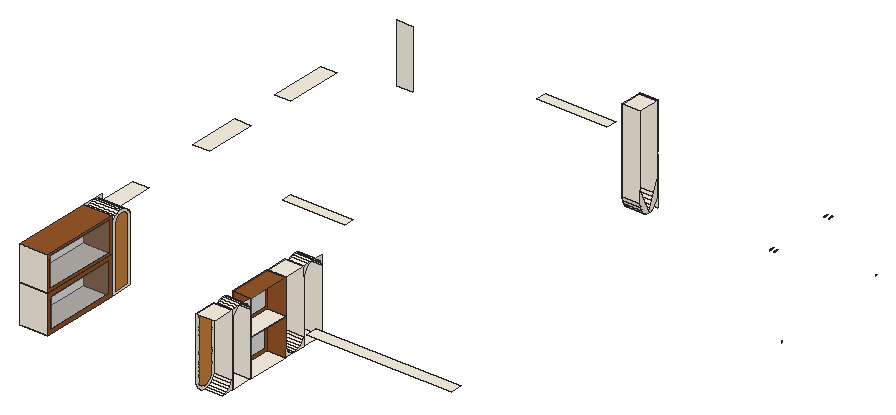
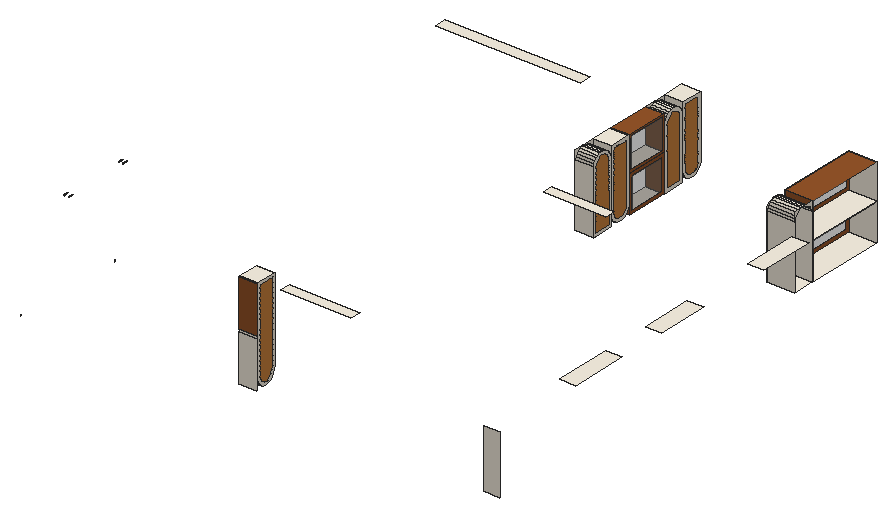
# SketchUp Ruby script. Lengths in inches.
U = 1.inch
M = Sketchup.active_model
def pt(a) = Geom::Point3d.new(a.map { |v| v * U })
def face(e, loops, mat)
  f = e.add_face(loops[0].map { |a| pt(a) })
  loops[1..].each { |l| e.add_face(l.map { |a| pt(a) }).erase! }
  f.material = f.back_material = mat if mat
  f
end
# faces: each face lists its corners as indices into pts; further lists are holes
def faces(e, pts, list, mat = nil) = list.each { |f| face(e, (f[0].is_a?(Array) ? f : [f]).map { |l| l.map { |i| pts[i] } }, mat) }
# xy, xz, yz: faces in a plane at the given z, y or x. An outline is a flat list of corners, or four numbers for a rectangle; further outlines are holes
def ring(l) = l.size == 4 ? [[l[0], l[1]], [l[2], l[1]], [l[2], l[3]], [l[0], l[3]]] : l.each_slice(2).to_a
def flat(e, list, mat, &to3) = list.each { |f| face(e, (f[0].is_a?(Array) ? f : [f]).map { |l| ring(l).map { |u, v| to3.(u, v) } }, mat) }
def xy(e, z, list, mat = nil) = flat(e, list, mat) { |x, y| [x, y, z] }
def xz(e, y, list, mat = nil) = flat(e, list, mat) { |x, z| [x, y, z] }
def yz(e, x, list, mat = nil) = flat(e, list, mat) { |y, z| [x, y, z] }
def lines(e, pts, list) = list.each { |a, b| e.add_line(pt(pts[a]), pt(pts[b])) }
# prism: a flat outline (further loops are holes) pulled along v
def prism(e, loops, v, mat = nil)
  f = face(e, loops, mat); d = Geom::Vector3d.new(v.map { |x| x * U })
  f.pushpull(f.normal.samedirection?(d) ? d.length : -d.length)
end
def box(e, o, s, mat = nil) = prism(e, [[o, [o[0] + s[0], o[1], o[2]], [o[0] + s[0], o[1] + s[1], o[2]], [o[0], o[1] + s[1], o[2]]]], [0, 0, s[2]], mat)
def at(x, y, z, deg = 0) = Geom::Transformation.translation(pt([x, y, z])) * Geom::Transformation.rotation(ORIGIN, Z_AXIS, deg.degrees)
def axes(o, x, y, z) = Geom::Transformation.new([*x, 0, *y, 0, *z, 0, *pt(o).to_a, 1])
def part(name) = M.definitions.add(name)
# library, detail: a bought-in or finely detailed component or shape, given as its bounding box
def library(name, o, s) = part(name).tap { |d| box(d.entities, o, s) }
def detail(e, o, s) = box(e.add_group.entities, o, s)
def put(e, d, t, mat = nil) = e.add_instance(d, t).tap { |i| i.material = mat if mat }
def group(e, t, mat = nil) = e.add_group.tap { |g| g.transformation = t; g.material = mat if mat }.entities
root = M.entities
M.materials.add("Material \#0").color = [86, 53, 35]
M.materials.add("Material \#1").color = [140, 140, 140]
M.materials.add("[0030_OldLace]").color = [253, 245, 230]
M.materials.add("[0040_Peru]").color = [205, 133, 63]
M.materials.add("[Translucent Glass Gray]").color = [128, 128, 128]
M.materials["[Translucent Glass Gray]"].alpha = 0.5
M.materials.add("[Wood Cherry Original]").color = [152, 86, 42]
c1 = part("3DGeom~17_Defintion")
yz(c1.entities,-1908.8,[[-436.03,-21.87,-436.73,-21.5,-435.91,-21.83],[436.03,-21.87,435.91,-21.83,436.73,-21.5],[-435.91,-21.83,-436.73,-21.5,-436.15,-21.125],[-435.91,-21.83,-436.15,-21.125,-435.87,-21.72],[435.91,-21.83,435.87,-21.72,436.15,-21.125],
  [435.91,-21.83,436.15,-21.125,436.73,-21.5],[-436.73,-21.5,-484.73,-21.37,-436.15,-1.11],[-471.46,-21.5,-484.73,-21.37,-436.73,-21.5],[-477.2,-21.5,-484.73,-21.37,-471.46,-21.5],[-481.82,-21.5,-484.73,-21.37,-477.2,-21.5],
  [-436.73,-21.5,-436.15,-1.11,-436.15,-21.125],[436.73,-21.5,436.15,-21.125,471.46,-21.5],[471.46,-21.5,436.15,-21.125,477.2,-21.5],[477.2,-21.5,436.15,-21.125,499.98,-0.85],[477.2,-21.5,499.98,-0.85,481.82,-21.5],
  [481.82,-21.5,487.35,-21,484.73,-21.37],[481.82,-21.5,491.8,-19.52,487.35,-21],[481.82,-21.5,497.64,-13.67,491.8,-19.52],[481.82,-21.5,499.98,-0.85,497.64,-13.67],[-484.73,-21.37,-498.5,-11.58,-499.84,-0.37],
  [-484.73,-21.37,-499.84,-0.37,-499.4,-0.5],[-484.73,-21.37,-499.4,-0.5,-436.15,-1.11],[-484.73,-21.37,-493.63,-18.42,-498.5,-11.58],[-484.73,-21.37,-489.71,-20.375,-493.63,-18.42],[-484.73,-21.37,-487.35,-21,-489.71,-20.375],
  [436.15,-21.125,436.15,-1.11,436.73,-0.74],[436.15,-21.125,436.73,-0.74,499.98,-0.85],[487.35,-21,491.8,-19.52,489.71,-20.375],[-489.71,-20.375,-491.8,-19.52,-493.63,-18.42],[491.8,-19.52,495.21,-17.08,493.63,-18.42],
  [491.8,-19.52,497.64,-13.67,495.21,-17.08],[-493.63,-18.42,-496.54,-15.5,-498.5,-11.58],[-493.63,-18.42,-495.21,-17.08,-496.54,-15.5],[495.21,-17.08,497.64,-13.67,496.54,-15.5],[-496.54,-15.5,-497.64,-13.67,-498.5,-11.58],
  [497.64,-13.67,499.125,-9.22,498.5,-11.58],[497.64,-13.67,499.625,-3.69,499.125,-9.22],[497.64,-13.67,499.98,-0.85,499.625,-3.69],[-498.5,-11.58,-499.625,-3.69,-499.84,-0.37],[-498.5,-11.58,-499.5,-6.6,-499.625,-3.69],
  [-498.5,-11.58,-499.125,-9.22,-499.5,-6.6],[499.125,-9.22,499.625,-3.69,499.5,-6.6],[-499.625,-3.69,-499.98,-0.85,-500,-0.52],[-499.625,-3.69,-500,-0.52,-499.84,-0.37],[-436.15,-1.11,-499.4,-0.5,-471.46,-0.74],
  [-436.15,-1.11,-471.46,-0.74,-436.73,-0.74],[-436.15,-1.11,-436.73,-0.74,-435.91,-0.41],[-436.15,-1.11,-435.91,-0.41,-435.87,-0.52],[436.15,-1.11,435.87,-0.52,435.91,-0.41],[436.15,-1.11,435.91,-0.41,436.73,-0.74],
  [499.98,-0.85,436.73,-0.74,471.46,-0.74],[499.98,-0.85,471.46,-0.74,499.4,-0.5],[499.98,-0.85,499.4,-0.5,499.96,-0.41],[499.98,-0.85,499.96,-0.41,500,-0.52],[-436.73,-0.74,-436.03,-0.37,-435.91,-0.41],
  [436.73,-0.74,435.91,-0.41,436.03,-0.37],[-500,-0.52,-499.96,-0.41,-499.84,-0.37],[499.4,-0.5,499.84,-0.37,499.96,-0.41],[-499.84,141.21,-499.96,141.25,-499.4,141.35],[-436.03,141.21,-436.73,141.59,-435.91,141.25],
  [436.03,141.21,435.91,141.25,436.73,141.59],[499.84,141.21,484.73,162.21,498.5,152.42],[499.84,141.21,499.4,141.35,484.73,162.21],[499.84,141.21,498.5,152.42,499.625,144.53],[499.84,141.21,499.625,144.53,500,141.37],
  [499.84,141.21,500,141.37,499.96,141.25],[-499.96,141.25,-500,141.37,-499.98,141.69],[-499.96,141.25,-499.98,141.69,-499.4,141.35],[-435.91,141.25,-436.73,141.59,-436.15,141.96],[-435.91,141.25,-436.15,141.96,-435.87,141.37],
  [435.91,141.25,435.87,141.37,436.15,141.96],[435.91,141.25,436.15,141.96,436.73,141.59],[-499.4,141.35,-499.98,141.69,-471.46,141.59],[499.4,141.35,436.15,141.96,484.73,162.21],[499.4,141.35,471.46,141.59,436.15,141.96],
  [500,141.37,499.625,144.53,499.98,141.69],[-436.73,141.59,-499.98,141.69,-436.15,161.97],[-471.46,141.59,-499.98,141.69,-436.73,141.59],[-436.73,141.59,-436.15,161.97,-436.15,141.96],[436.73,141.59,436.15,141.96,471.46,141.59],
  [-499.98,141.69,-477.2,162.34,-436.15,161.97],[-499.98,141.69,-481.82,162.34,-477.2,162.34],[-499.98,141.69,-497.64,154.51,-481.82,162.34],[-499.98,141.69,-499.625,144.53,-497.64,154.51],[436.15,141.96,436.15,161.97,436.73,162.34],
  [436.15,141.96,436.73,162.34,484.73,162.21],[-499.625,144.53,-499.125,150.07,-497.64,154.51],[-499.625,144.53,-499.5,147.44,-499.125,150.07],[499.625,144.53,498.5,152.42,499.5,147.44],[499.5,147.44,498.5,152.42,499.125,150.07],
  [-499.125,150.07,-498.5,152.42,-497.64,154.51],[498.5,152.42,484.73,162.21,493.63,159.26],[498.5,152.42,493.63,159.26,496.54,156.34],[498.5,152.42,496.54,156.34,497.64,154.51],[-497.64,154.51,-491.8,160.36,-481.82,162.34],
  [-497.64,154.51,-495.21,157.92,-491.8,160.36],[-497.64,154.51,-496.54,156.34,-495.21,157.92],[496.54,156.34,493.63,159.26,495.21,157.92],[-495.21,157.92,-493.63,159.26,-491.8,160.36],[493.63,159.26,484.73,162.21,489.71,161.22],
  [493.63,159.26,489.71,161.22,491.8,160.36],[-491.8,160.36,-487.35,161.84,-481.82,162.34],[-491.8,160.36,-489.71,161.22,-487.35,161.84],[489.71,161.22,484.73,162.21,487.35,161.84],[-487.35,161.84,-484.73,162.21,-481.82,162.34],
  [-436.15,161.97,-477.2,162.34,-471.46,162.34],[-436.15,161.97,-471.46,162.34,-436.73,162.34],[-436.15,161.97,-436.73,162.34,-435.91,162.68],[-436.15,161.97,-435.91,162.68,-435.87,162.56],[436.15,161.97,435.87,162.56,435.91,162.68],
  [436.15,161.97,435.91,162.68,436.73,162.34],[484.73,162.21,436.73,162.34,471.46,162.34],[484.73,162.21,471.46,162.34,477.2,162.34],[484.73,162.21,477.2,162.34,481.82,162.34],[-436.73,162.34,-436.03,162.72,-435.91,162.68],
  [436.73,162.34,435.91,162.68,436.03,162.72]],"Material \#0")
xy(root,67.4375,[[9,54.465,24.375,98.59],[9,99.09,24.375,111.09]],"[0030_OldLace]")
xy(root,67.8125,[[106.9375,66.277,117,78.277],[106.9375,78.777,117,102.777],[106.9375,115.777,117,127.777]],"[0030_OldLace]")
xy(root,87.875,[[9,54.465,24.375,98.59]],"[Wood Cherry Original]")
xy(root,88.125,[[106.9375,78.777,117,102.777]],"[Wood Cherry Original]")
xy(root,88.375,[[9,54.465,24.375,98.59]],"[0030_OldLace]")
xy(root,88.625,[[106.9375,78.777,117,102.777]],"[0030_OldLace]")
xy(root,96,[[0,112.59,9,143.465],[0,185.34,9,214.09],[0,241.59,9,273.527]],"[0030_OldLace]")
xy(root,106,[[153.875,71.465,234.432,77.465],[71.67,157.465,106.375,162.902],[102,295.465,140.9375,301.465]],"[0030_OldLace]")
xy(root,107.5625,[[9,54.465,24.375,98.59]],"[Wood Cherry Original]")
xy(root,107.6875,[[106.9375,53.777,117,65.777],[106.9375,103.277,117,115.277]],"[0030_OldLace]")
xy(root,107.6875,[[106.9375,78.777,117,102.777]],"[Wood Cherry Original]")
xy(root,114.625,[[143,302.965,153,314.965]],"[0030_OldLace]")
xz(root,54.465,[[9,67.4375,24.375,87.875],[9,88.375,24.375,107.5625]],"[0030_OldLace]")
xz(root,65.777,[[106.9375,72.8125,117,107.6875]],"[0030_OldLace]")
xz(root,66.277,[[106.9375,67.8125,117,102.6875]],"[0030_OldLace]")
xz(root,78.277,[[106.9375,67.8125,117,102.6875]],"[0030_OldLace]")
xz(root,78.777,[[106.9375,67.8125,117,88.125],[106.9375,88.625,117,107.6875]],"[Wood Cherry Original]")
xz(root,98.59,[[9,67.4375,24.375,87.875],[9,88.375,24.375,107.5625]],"[Wood Cherry Original]")
xz(root,99.09,[[9,67.4375,24.375,102.5625]],"[0030_OldLace]")
xz(root,102.777,[[106.9375,67.8125,117,88.125],[106.9375,88.625,117,107.6875]],"[Wood Cherry Original]")
xz(root,103.277,[[106.9375,72.8125,117,107.6875]],"[0030_OldLace]")
xz(root,111.09,[[9,67.4375,24.375,102.5625]],"[0030_OldLace]")
xz(root,115.277,[[106.9375,72.8125,117,107.6875]],"[0030_OldLace]")
xz(root,115.777,[[106.9375,67.8125,117,102.6875]],"[0030_OldLace]")
xz(root,127.777,[[106.9375,67.8125,117,102.6875]],"[0030_OldLace]")
xz(root,302.965,[[143,68.556,153,114.625]],"[0030_OldLace]")
xz(root,314.965,[[143,68.556,153,114.625]],"[0030_OldLace]")
xz(root,315.465,[[143,61.536,153,87.422]],"[0030_OldLace]")
xz(root,315.465,[[143,88.826,153,114.625]],"[Wood Cherry Original]")
xz(root,326.027,[[0,63.5,9,96]],"[0030_OldLace]")
yz(root,9,[[99.09,102.5625,99.503,103.91,100.213,105.127,101.185,106.149,102.365,106.92,103.69,107.4,105.09,107.5625,99.09,107.5625],[111.09,102.5625,111.09,107.5625,105.09,107.5625,106.49,107.4,107.815,106.92,108.995,106.149,109.966,105.127,110.677,103.91]],"[0030_OldLace]")
yz(root,24.375,[[[99.09,67.4375,111.09,67.4375,111.09,102.5625,110.677,103.91,109.966,105.127,108.995,106.149,107.815,106.92,106.49,107.4,105.09,107.5625,103.69,107.4,102.365,106.92,101.185,106.149,100.213,105.127,99.503,103.91,99.09,102.5625],[100.282,68.63,100.282,102.384,100.602,103.429,101.173,104.406,101.953,105.227,102.901,105.846,103.965,106.232,105.09,106.362,106.215,106.232,107.279,105.846,108.227,105.227,109.007,104.406,109.578,103.429,109.898,102.384,109.898,68.63]]],"[0030_OldLace]")
yz(root,24.375,[[100.282,68.63,109.898,68.63,109.898,102.384,109.578,103.429,109.007,104.406,108.227,105.227,107.279,105.846,106.215,106.232,105.09,106.362,103.965,106.232,102.901,105.846,101.953,105.227,101.173,104.406,100.602,103.429,100.282,102.384]],"[0040_Peru]")
yz(root,24.375,[[56.357,69.33,96.697,85.983],[55.951,89.861,97.104,106.077]],"[Translucent Glass Gray]")
yz(root,24.375,[[[54.465,67.4375,98.59,87.875],[56.357,69.33,96.697,85.983]],[[54.465,88.375,98.59,107.5625],[55.951,89.861,97.104,106.077]]],"[Wood Cherry Original]")
yz(root,106.9375,[[[59.777,67.8125,58.377,67.975,57.052,68.455,55.872,69.226,54.901,70.248,54.19,71.465,53.777,72.8125,53.777,107.6875,65.777,107.6875,65.777,72.8125,65.365,71.465,64.654,70.248,63.683,69.226,62.503,68.455,61.177,67.975],[59.777,69.279,60.841,69.403,61.847,69.768,62.743,70.353,63.481,71.129,64.021,72.053,64.32,73.031,64.32,106.23,55.235,106.23,55.235,73.031,55.534,72.053,56.074,71.129,56.811,70.353,57.707,69.768,58.714,69.403]],[[66.277,67.8125,66.277,102.6875,66.69,104.035,67.401,105.252,68.372,106.274,69.552,107.045,70.877,107.525,72.277,107.6875,73.677,107.525,75.003,107.045,76.183,106.274,77.154,105.252,77.865,104.035,78.277,102.6875,78.277,67.8125],[67.924,69.459,76.631,69.459,76.631,102.441,76.346,103.37,75.828,104.256,75.121,105,74.262,105.562,73.297,105.911,72.277,106.03,71.258,105.911,70.293,105.562,69.434,105,68.726,104.256,68.209,103.37,67.924,102.441]],[[109.277,67.8125,107.877,67.975,106.552,68.455,105.372,69.226,104.401,70.248,103.69,71.465,103.277,72.8125,103.277,107.6875,115.277,107.6875,115.277,72.8125,114.865,71.465,114.154,70.248,113.183,69.226,112.003,68.455,110.677,67.975],[109.277,69.662,110.253,69.776,111.176,70.11,111.998,70.648,112.675,71.359,113.17,72.207,113.44,73.088,113.44,105.85,105.115,105.85,105.115,73.088,105.384,72.207,105.88,71.359,106.557,70.648,107.379,70.11,108.302,69.776]],[[115.777,67.8125,115.777,102.6875,116.19,104.035,116.901,105.252,117.872,106.274,119.052,107.045,120.377,107.525,121.777,107.6875,123.177,107.525,124.503,107.045,125.683,106.274,126.654,105.252,127.365,104.035,127.777,102.6875,127.777,67.8125],[117.355,69.39,126.2,69.39,126.2,102.451,125.91,103.398,125.384,104.298,124.666,105.054,123.793,105.624,122.813,105.979,121.777,106.1,120.742,105.979,119.761,105.624,118.889,105.054,118.17,104.298,117.644,103.398,117.355,102.451]]],"[0030_OldLace]")
yz(root,106.9375,[[59.777,69.279,58.714,69.403,57.707,69.768,56.811,70.353,56.074,71.129,55.534,72.053,55.235,73.031,55.235,106.23,64.32,106.23,64.32,73.031,64.021,72.053,63.481,71.129,62.743,70.353,61.847,69.768,60.841,69.403],[117.355,69.39,117.355,102.451,117.644,103.398,118.17,104.298,118.889,105.054,119.761,105.624,120.742,105.979,121.777,106.1,122.813,105.979,123.793,105.624,124.666,105.054,125.384,104.298,125.91,103.398,126.2,102.451,126.2,69.39],[67.924,69.459,67.924,102.441,68.209,103.37,68.726,104.256,69.434,105,70.293,105.562,71.258,105.911,72.277,106.03,73.297,105.911,74.262,105.562,75.121,105,75.828,104.256,76.346,103.37,76.631,102.441,76.631,69.459],[109.277,69.662,108.302,69.776,107.379,70.11,106.557,70.648,105.88,71.359,105.384,72.207,105.115,73.088,105.115,105.85,113.44,105.85,113.44,73.088,113.17,72.207,112.675,71.359,111.998,70.648,111.176,70.11,110.253,69.776]],"[0040_Peru]")
yz(root,106.9375,[[80.288,69.323,101.267,86.614],[79.813,89.661,101.741,106.651]],"[Translucent Glass Gray]")
yz(root,106.9375,[[[78.777,67.8125,102.777,88.125],[80.288,69.323,101.267,86.614]],[[78.777,88.625,102.777,107.6875],[79.813,89.661,101.741,106.651]]],"[Wood Cherry Original]")
yz(root,117,[[59.777,67.8125,61.177,67.975,62.503,68.455,63.683,69.226,64.654,70.248,65.365,71.465,65.777,72.8125,65.777,67.8125],[103.277,67.8125,103.277,72.8125,103.69,71.465,104.401,70.248,105.372,69.226,106.552,68.455,107.877,67.975,109.277,67.8125],[109.277,67.8125,110.677,67.975,112.003,68.455,113.183,69.226,114.154,70.248,114.865,71.465,115.277,72.8125,115.277,67.8125],[66.277,102.6875,66.277,107.6875,72.277,107.6875,70.877,107.525,69.552,107.045,68.372,106.274,67.401,105.252,66.69,104.035],[78.277,102.6875,77.865,104.035,77.154,105.252,76.183,106.274,75.003,107.045,73.677,107.525,72.277,107.6875,78.277,107.6875],
  [115.777,102.6875,115.777,107.6875,121.777,107.6875,120.377,107.525,119.052,107.045,117.872,106.274,116.901,105.252,116.19,104.035],[127.777,102.6875,127.365,104.035,126.654,105.252,125.683,106.274,124.503,107.045,123.177,107.525,121.777,107.6875,127.777,107.6875]],"[0030_OldLace]")
yz(root,143,[[[308.965,61.536,307.565,61.765,306.24,62.439,305.06,63.521,304.088,64.955,303.378,66.664,302.965,68.556,302.965,114.625,314.965,114.625,314.965,68.556,314.552,66.664,313.841,64.955,312.87,63.521,311.69,62.439,310.365,61.765],[308.965,63.097,309.88,63.246,310.804,63.716,311.696,64.534,312.479,65.69,313.077,67.128,313.425,68.722,313.425,113.085,304.505,113.085,304.505,68.722,304.853,67.128,305.451,65.69,306.234,64.534,307.125,63.716,308.049,63.246]]],"[0030_OldLace]")
yz(root,143,[[308.965,63.097,308.049,63.246,307.125,63.716,306.234,64.534,305.451,65.69,304.853,67.128,304.505,68.722,304.505,113.085,313.425,113.085,313.425,68.722,313.077,67.128,312.479,65.69,311.696,64.534,310.804,63.716,309.88,63.246]],"[0040_Peru]")
yz(root,153,[[308.965,61.536,307.565,61.765,306.24,62.439,305.06,63.521,304.088,64.955,303.378,66.664,302.965,68.556,302.965,75.3],[308.965,61.536,314.965,75.3,314.965,68.556,314.552,66.664,313.841,64.955,312.87,63.521,311.69,62.439,310.365,61.765]],"[0030_OldLace]")
yz(root,263.952,[[327.532,61.352,327.521,61.353,327.543,61.512],[327.521,61.353,327.532,61.514,327.543,61.512],[327.543,61.512,327.532,61.514,327.573,61.656],[327.532,61.514,327.5625,61.661,327.573,61.656],[327.573,61.656,327.5625,61.661,327.624,61.795],
  [327.5625,61.661,327.614,61.803,327.624,61.795],[327.624,61.795,327.614,61.803,327.684,61.907]],"Material \#1")
yz(root,264.101,[[327.532,61.352,327.543,61.512,327.521,61.353],[327.521,61.353,327.543,61.512,327.532,61.514],[327.543,61.512,327.573,61.656,327.532,61.514],[327.532,61.514,327.573,61.656,327.5625,61.661],[327.573,61.656,327.624,61.795,327.5625,61.661],
  [327.5625,61.661,327.624,61.795,327.614,61.803],[327.624,61.795,327.684,61.907,327.614,61.803],[327.614,61.803,327.684,61.907,327.676,61.917]],"Material \#1")
yz(root,265.622,[[260.515,58.184,260.463,58.193,260.465,58.202],[260.515,58.184,260.465,58.202,260.515,58.194],[260.515,58.184,260.515,58.194,260.567,58.193],[260.463,58.193,260.415,58.219,260.418,58.228],[260.463,58.193,260.418,58.228,260.465,58.202],
  [260.567,58.193,260.515,58.194,260.565,58.202],[260.567,58.193,260.565,58.202,260.615,58.219],[260.565,58.202,260.611,58.228,260.615,58.219],[260.415,58.219,260.373,58.261,260.378,58.268],[260.415,58.219,260.378,58.268,260.418,58.228],
  [260.615,58.219,260.611,58.228,260.657,58.261],[260.611,58.228,260.651,58.268,260.657,58.261],[260.373,58.261,260.341,58.316,260.348,58.321],[260.373,58.261,260.348,58.321,260.378,58.268],[260.657,58.261,260.651,58.268,260.688,58.316],
  [260.651,58.268,260.682,58.321,260.688,58.316],[260.341,58.316,260.321,58.38,260.328,58.383],[260.341,58.316,260.328,58.383,260.348,58.321],[260.688,58.316,260.682,58.321,260.708,58.38],[260.682,58.321,260.701,58.383,260.708,58.38],
  [260.321,58.38,260.314,58.449,260.322,58.449],[260.321,58.38,260.322,58.449,260.328,58.383],[260.708,58.38,260.701,58.383,260.715,58.449],[260.701,58.383,260.708,58.449,260.715,58.449],[260.314,58.449,260.321,58.517,260.328,58.515],
  [260.314,58.449,260.328,58.515,260.322,58.449],[260.708,58.449,260.701,58.515,260.708,58.517],[260.708,58.449,260.708,58.517,260.715,58.449],[260.328,58.515,260.321,58.517,260.348,58.576],[260.701,58.515,260.682,58.576,260.688,58.581],
  [260.701,58.515,260.688,58.581,260.708,58.517],[260.321,58.517,260.341,58.581,260.348,58.576],[260.348,58.576,260.341,58.581,260.378,58.629],[260.682,58.576,260.651,58.629,260.657,58.636],[260.682,58.576,260.657,58.636,260.688,58.581],
  [260.341,58.581,260.373,58.636,260.378,58.629],[260.378,58.629,260.373,58.636,260.418,58.669],[260.651,58.629,260.611,58.669,260.615,58.678],[260.651,58.629,260.615,58.678,260.657,58.636],[260.373,58.636,260.415,58.678,260.418,58.669],
  [260.418,58.669,260.415,58.678,260.465,58.695],[260.611,58.669,260.565,58.695,260.567,58.704],[260.611,58.669,260.567,58.704,260.615,58.678],[260.415,58.678,260.463,58.704,260.465,58.695],[260.465,58.695,260.463,58.704,260.515,58.703],
  [260.565,58.695,260.515,58.703,260.515,58.713],[260.565,58.695,260.515,58.713,260.567,58.704],[260.515,58.703,260.463,58.704,260.515,58.713]],"Material \#1")
yz(root,265.627,[[260.316,58.238,260.262,58.493,260.296,58.381],[260.316,58.238,260.267,58.371,260.262,58.493],[260.316,58.238,260.286,58.301,260.267,58.371],[260.296,58.381,260.262,58.493,260.29,58.449],[260.29,58.449,260.262,58.493,260.296,58.517],
  [260.262,58.493,260.279,58.577,260.311,58.65],[260.262,58.493,260.311,58.65,260.36,58.716],[260.262,58.493,260.3125,58.579,260.296,58.517],[260.262,58.493,260.339,58.634,260.3125,58.579],[260.262,58.493,260.36,58.716,260.364,58.722],
  [260.262,58.493,260.364,58.722,260.367,58.728],[260.279,58.577,260.293,58.615,260.311,58.65],[260.311,58.65,260.331,58.682,260.355,58.71],[260.311,58.65,260.355,58.71,260.36,58.716],[260.372,58.75,260.372,58.757,260.404,59.235],
  [260.372,58.757,260.372,59.117,260.376,59.16],[260.372,58.757,260.376,59.16,260.404,59.235],[260.376,59.16,260.387,59.2,260.404,59.235],[260.404,59.235,260.426,59.264,260.452,59.286]],"Material \#1")
p = [[153,308.965,61.536],[153,307.565,61.765],[143,307.565,61.765],[143,308.965,61.536],[153,310.365,61.765],[143,310.365,61.765],
  [153,306.24,62.439],[143,306.24,62.439],[153,311.69,62.439],[143,311.69,62.439],[153,305.06,63.521],[143,305.06,63.521],
  [153,312.87,63.521],[143,312.87,63.521],[153,304.088,64.955],[143,304.088,64.955],[153,313.841,64.955],[143,313.841,64.955],
  [153,303.378,66.664],[143,303.378,66.664],[153,314.552,66.664],[143,314.552,66.664],[153,302.965,68.556],[143,302.965,68.556],
  [153,314.965,68.556],[143,314.965,68.556],[117,61.177,67.975],[117,59.777,67.8125],[106.9375,59.777,67.8125],[106.9375,61.177,67.975],
  [117,109.277,67.8125],[117,107.877,67.975],[106.9375,107.877,67.975],[106.9375,109.277,67.8125],[117,110.677,67.975],[106.9375,110.677,67.975],
  [117,62.503,68.455],[106.9375,62.503,68.455],[117,106.552,68.455],[106.9375,106.552,68.455],[117,112.003,68.455],[106.9375,112.003,68.455],
  [117,63.683,69.226],[106.9375,63.683,69.226],[117,105.372,69.226],[106.9375,105.372,69.226],[117,113.183,69.226],[106.9375,113.183,69.226],
  [117,64.654,70.248],[106.9375,64.654,70.248],[117,104.401,70.248],[106.9375,104.401,70.248],[117,114.154,70.248],[106.9375,114.154,70.248],
  [117,65.365,71.465],[106.9375,65.365,71.465],[117,103.69,71.465],[106.9375,103.69,71.465],[117,114.865,71.465],[106.9375,114.865,71.465],
  [117,65.777,72.8125],[106.9375,65.777,72.8125],[117,103.277,72.8125],[106.9375,103.277,72.8125],[117,115.277,72.8125],[106.9375,115.277,72.8125],
  [9,99.503,103.91],[9,99.09,102.5625],[24.375,99.09,102.5625],[24.375,99.503,103.91],[9,111.09,102.5625],[9,110.677,103.91],
  [24.375,110.677,103.91],[24.375,111.09,102.5625],[117,66.277,102.6875],[117,66.69,104.035],[106.9375,66.69,104.035],[106.9375,66.277,102.6875],
  [117,77.865,104.035],[117,78.277,102.6875],[106.9375,78.277,102.6875],[106.9375,77.865,104.035],[117,115.777,102.6875],[117,116.19,104.035],
  [106.9375,116.19,104.035],[106.9375,115.777,102.6875],[117,127.365,104.035],[117,127.777,102.6875],[106.9375,127.777,102.6875],[106.9375,127.365,104.035],
  [9,100.213,105.127],[24.375,100.213,105.127],[9,109.966,105.127],[24.375,109.966,105.127],[117,67.401,105.252],[106.9375,67.401,105.252],
  [117,77.154,105.252],[106.9375,77.154,105.252],[117,116.901,105.252],[106.9375,116.901,105.252],[117,126.654,105.252],[106.9375,126.654,105.252],
  [9,101.185,106.149],[24.375,101.185,106.149],[9,108.995,106.149],[24.375,108.995,106.149],[117,68.372,106.274],[106.9375,68.372,106.274],
  [117,76.183,106.274],[106.9375,76.183,106.274],[117,117.872,106.274],[106.9375,117.872,106.274],[117,125.683,106.274],[106.9375,125.683,106.274],
  [9,102.365,106.92],[24.375,102.365,106.92],[9,107.815,106.92],[24.375,107.815,106.92],[117,69.552,107.045],[106.9375,69.552,107.045],
  [117,75.003,107.045],[106.9375,75.003,107.045],[117,119.052,107.045],[106.9375,119.052,107.045],[117,124.503,107.045],[106.9375,124.503,107.045],
  [9,103.69,107.4],[24.375,103.69,107.4],[9,106.49,107.4],[24.375,106.49,107.4],[117,70.877,107.525],[106.9375,70.877,107.525],
  [117,73.677,107.525],[106.9375,73.677,107.525],[117,120.377,107.525],[106.9375,120.377,107.525],[117,123.177,107.525],[106.9375,123.177,107.525],
  [9,105.09,107.5625],[24.375,105.09,107.5625],[117,72.277,107.6875],[106.9375,72.277,107.6875],[117,121.777,107.6875],[106.9375,121.777,107.6875],
  [153.875,77.465,106],[153.875,78.027,106]]
faces(root,p,[[0,1,2,3],[4,0,3,5],[1,6,7,2],[8,4,5,9],[6,10,11,7],[12,8,9,13],[10,14,15,11],[16,12,13,17],
  [14,18,19,15],[20,16,17,21],[18,22,23,19],[24,20,21,25],[26,27,28,29],[30,31,32,33],[34,30,33,35],[36,26,29,37],
  [31,38,39,32],[40,34,35,41],[42,36,37,43],[38,44,45,39],[46,40,41,47],[48,42,43,49],[44,50,51,45],[52,46,47,53],
  [54,48,49,55],[50,56,57,51],[58,52,53,59],[60,54,55,61],[56,62,63,57],[64,58,59,65],[66,67,68,69],[70,71,72,73],
  [74,75,76,77],[78,79,80,81],[82,83,84,85],[86,87,88,89],[90,66,69,91],[71,92,93,72],[75,94,95,76],[96,78,81,97],
  [83,98,99,84],[100,86,89,101],[102,90,91,103],[92,104,105,93],[94,106,107,95],[108,96,97,109],[98,110,111,99],[112,100,101,113],
  [114,102,103,115],[104,116,117,105],[106,118,119,107],[120,108,109,121],[110,122,123,111],[124,112,113,125],[126,114,115,127],[116,128,129,117],
  [118,130,131,119],[132,120,121,133],[122,134,135,123],[136,124,125,137],[138,126,127,139],[128,138,139,129],[130,140,141,131],[140,132,133,141],
  [134,142,143,135],[142,136,137,143]],"[0030_OldLace]")
lines(root,p,[[144,145]])
put(root,c1,axes([263.98,274.39,3.96],[0,0,-0.05346],[0,0.04046,0],[0.01534,0,0]),"Material \#0")
